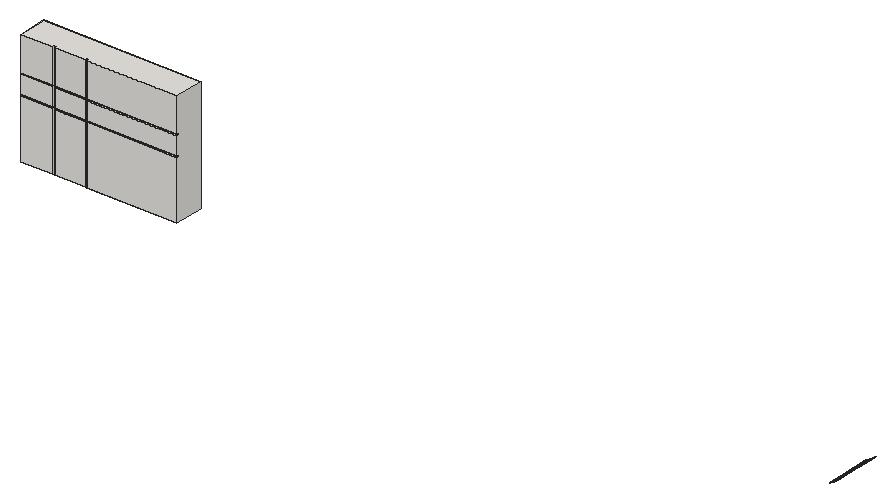
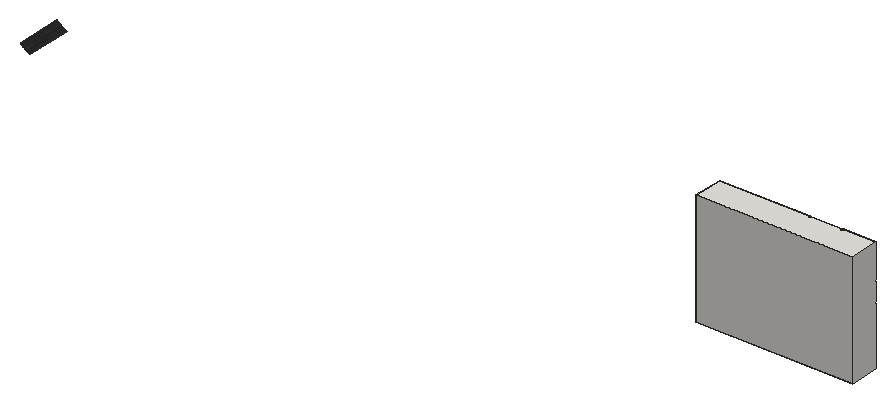
# SketchUp Ruby script. Lengths in inches.
U = 1.inch
M = Sketchup.active_model
def pt(a) = Geom::Point3d.new(a.map { |v| v * U })
def face(e, loops, mat)
  f = e.add_face(loops[0].map { |a| pt(a) })
  loops[1..].each { |l| e.add_face(l.map { |a| pt(a) }).erase! }
  f.material = f.back_material = mat if mat
  f
end
# faces: each face lists its corners as indices into pts; further lists are holes
def faces(e, pts, list, mat = nil) = list.each { |f| face(e, (f[0].is_a?(Array) ? f : [f]).map { |l| l.map { |i| pts[i] } }, mat) }
# xy, xz, yz: faces in a plane at the given z, y or x. An outline is a flat list of corners, or four numbers for a rectangle; further outlines are holes
def ring(l) = l.size == 4 ? [[l[0], l[1]], [l[2], l[1]], [l[2], l[3]], [l[0], l[3]]] : l.each_slice(2).to_a
def flat(e, list, mat, &to3) = list.each { |f| face(e, (f[0].is_a?(Array) ? f : [f]).map { |l| ring(l).map { |u, v| to3.(u, v) } }, mat) }
def xy(e, z, list, mat = nil) = flat(e, list, mat) { |x, y| [x, y, z] }
def xz(e, y, list, mat = nil) = flat(e, list, mat) { |x, z| [x, y, z] }
def yz(e, x, list, mat = nil) = flat(e, list, mat) { |y, z| [x, y, z] }
def lines(e, pts, list) = list.each { |a, b| e.add_line(pt(pts[a]), pt(pts[b])) }
# prism: a flat outline (further loops are holes) pulled along v
def prism(e, loops, v, mat = nil)
  f = face(e, loops, mat); d = Geom::Vector3d.new(v.map { |x| x * U })
  f.pushpull(f.normal.samedirection?(d) ? d.length : -d.length)
end
def box(e, o, s, mat = nil) = prism(e, [[o, [o[0] + s[0], o[1], o[2]], [o[0] + s[0], o[1] + s[1], o[2]], [o[0], o[1] + s[1], o[2]]]], [0, 0, s[2]], mat)
def at(x, y, z, deg = 0) = Geom::Transformation.translation(pt([x, y, z])) * Geom::Transformation.rotation(ORIGIN, Z_AXIS, deg.degrees)
def axes(o, x, y, z) = Geom::Transformation.new([*x, 0, *y, 0, *z, 0, *pt(o).to_a, 1])
def part(name) = M.definitions.add(name)
# library, detail: a bought-in or finely detailed component or shape, given as its bounding box
def library(name, o, s) = part(name).tap { |d| box(d.entities, o, s) }
def detail(e, o, s) = box(e.add_group.entities, o, s)
def put(e, d, t, mat = nil) = e.add_instance(d, t).tap { |i| i.material = mat if mat }
def group(e, t, mat = nil) = e.add_group.tap { |g| g.transformation = t; g.material = mat if mat }.entities
root = M.entities
M.materials.add("1496 AP 8293 CARBON COPY").color = [58, 58, 58]
M.materials.add("[Carrera Marble]").color = [233, 230, 225]
p = [[299.59,71,145.18],[299.8,71,145.3],[299.8,85,145.3],[299.59,85,145.18],[300,71,145.41],[300,85,145.41],
  [300.2,71,145.53],[300.2,85,145.53],[300.4,71,145.65],[300.4,85,145.65],[300.61,71,145.78],[300.61,85,145.78],
  [300.8,71,145.9],[300.8,85,145.9],[301,71,146.03],[301,85,146.03],[301.2,71,146.17],[301.2,85,146.17],
  [301.39,71,146.3],[301.39,85,146.3],[301.58,71,146.4375],[301.58,85,146.4375],[301.77,71,146.58],[301.77,85,146.58],
  [301.96,71,146.72],[301.96,85,146.72],[302.14,71,146.86],[302.14,85,146.86],[302.33,71,147.01],[302.33,85,147.01],
  [302.51,71,147.16],[302.51,85,147.16],[302.69,71,147.3125],[302.69,85,147.3125]]
faces(root,p,[[0,1,2,3],[1,4,5,2],[4,6,7,5],[6,8,9,7],[8,10,11,9],[10,12,13,11],[12,14,15,13],[14,16,17,15],
  [16,18,19,17],[18,20,21,19],[20,22,23,21],[22,24,25,23],[24,26,27,25],[26,28,29,27],[28,30,31,29],[30,32,33,31]],"1496 AP 8293 CARBON COPY")
g1 = group(root,at(47,75.5,143),"[Carrera Marble]")
xy(g1,0,[[0,0,0,9,48.23,9,48.23,0,20.5,0,20.5,0.5,20,0.5,20,0,10.5,0,10.5,0.5,10,0.5,10,0]])
xy(g1,18,[[0,0,10,0.5],[10.5,0,20,0.5],[20.5,0,48.23,0.5]])
xy(g1,18.5,[[0,0,10,0.5],[10.5,0,20,0.5],[20.5,0,48.23,0.5]])
xy(g1,24,[[0,0,10,0.5],[10.5,0,20,0.5],[20.5,0,48.23,0.5]])
xy(g1,24.5,[[0,0,10,0.5],[10.5,0,20,0.5],[20.5,0,48.23,0.5]])
xy(g1,35,[[0,0,10,0,10,0.5,10.5,0.5,10.5,0,20,0,20,0.5,20.5,0.5,20.5,0,48.23,0,48.23,9,0,9]])
xz(g1,0,[[0,0,10,18],[10.5,0,20,18],[20.5,0,48.23,18],[0,18.5,10,24],[10.5,18.5,20,24],
  [20.5,18.5,48.23,24],[0,24.5,10,35],[10.5,24.5,20,35],[20.5,24.5,48.23,35]])
xz(g1,0.5,[[[10,0,10.5,0,10.5,18,20,18,20,0,20.5,0,20.5,18,48.23,18,48.23,18.5,20.5,18.5,20.5,24,48.23,24,48.23,24.5,20.5,24.5,20.5,35,20,35,20,24.5,10.5,24.5,10.5,35,10,35,10,24.5,0,24.5,0,24,10,24,10,18.5,0,18.5,0,18,10,18],[10.5,18.5,20,24]]])
xz(g1,9,[[0,0,48.23,35]])
yz(g1,0,[[0,0,0,18,0.5,18,0.5,18.5,0,18.5,0,24,0.5,24,0.5,24.5,0,24.5,0,35,9,35,9,0]])
yz(g1,10,[[0,0,0.5,18],[0,18.5,0.5,24],[0,24.5,0.5,35]])
yz(g1,10.5,[[0,0,0.5,18],[0,18.5,0.5,24],[0,24.5,0.5,35]])
yz(g1,20,[[0,0,0.5,18],[0,18.5,0.5,24],[0,24.5,0.5,35]])
yz(g1,20.5,[[0,0,0.5,18],[0,18.5,0.5,24],[0,24.5,0.5,35]])
yz(g1,48.23,[[0,0,9,0,9,35,0,35,0,24.5,0.5,24.5,0.5,24,0,24,0,18.5,0.5,18.5,0.5,18,0,18]])
